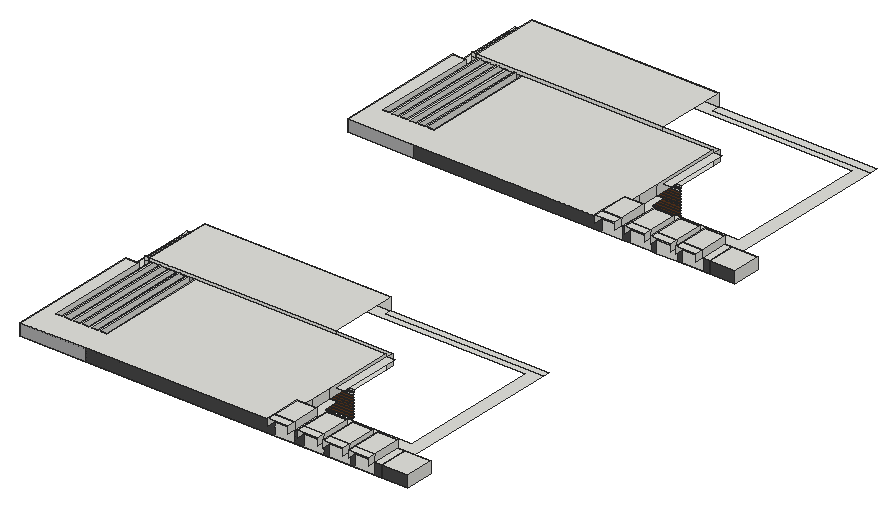
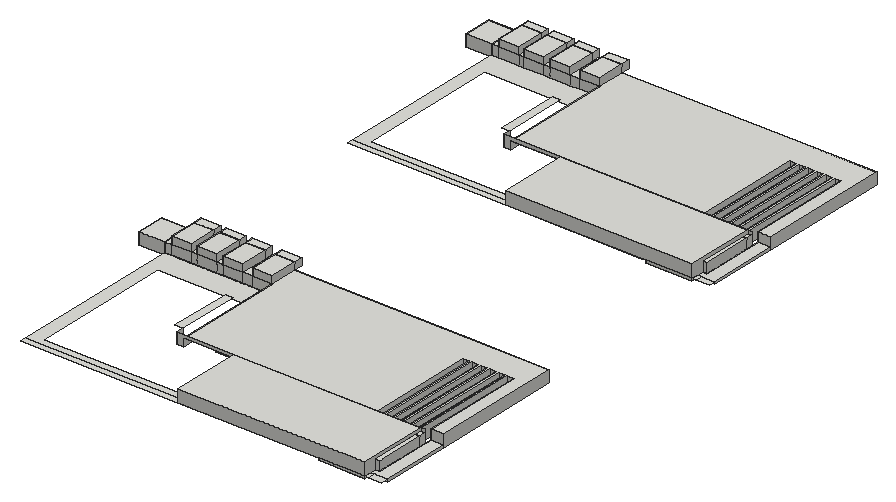
# SketchUp Ruby script. Lengths in inches.
U = 1.inch
M = Sketchup.active_model
def pt(a) = Geom::Point3d.new(a.map { |v| v * U })
def face(e, loops, mat)
  f = e.add_face(loops[0].map { |a| pt(a) })
  loops[1..].each { |l| e.add_face(l.map { |a| pt(a) }).erase! }
  f.material = f.back_material = mat if mat
  f
end
# faces: each face lists its corners as indices into pts; further lists are holes
def faces(e, pts, list, mat = nil) = list.each { |f| face(e, (f[0].is_a?(Array) ? f : [f]).map { |l| l.map { |i| pts[i] } }, mat) }
# xy, xz, yz: faces in a plane at the given z, y or x. An outline is a flat list of corners, or four numbers for a rectangle; further outlines are holes
def ring(l) = l.size == 4 ? [[l[0], l[1]], [l[2], l[1]], [l[2], l[3]], [l[0], l[3]]] : l.each_slice(2).to_a
def flat(e, list, mat, &to3) = list.each { |f| face(e, (f[0].is_a?(Array) ? f : [f]).map { |l| ring(l).map { |u, v| to3.(u, v) } }, mat) }
def xy(e, z, list, mat = nil) = flat(e, list, mat) { |x, y| [x, y, z] }
def xz(e, y, list, mat = nil) = flat(e, list, mat) { |x, z| [x, y, z] }
def yz(e, x, list, mat = nil) = flat(e, list, mat) { |y, z| [x, y, z] }
def lines(e, pts, list) = list.each { |a, b| e.add_line(pt(pts[a]), pt(pts[b])) }
# prism: a flat outline (further loops are holes) pulled along v
def prism(e, loops, v, mat = nil)
  f = face(e, loops, mat); d = Geom::Vector3d.new(v.map { |x| x * U })
  f.pushpull(f.normal.samedirection?(d) ? d.length : -d.length)
end
def box(e, o, s, mat = nil) = prism(e, [[o, [o[0] + s[0], o[1], o[2]], [o[0] + s[0], o[1] + s[1], o[2]], [o[0], o[1] + s[1], o[2]]]], [0, 0, s[2]], mat)
def at(x, y, z, deg = 0) = Geom::Transformation.translation(pt([x, y, z])) * Geom::Transformation.rotation(ORIGIN, Z_AXIS, deg.degrees)
def axes(o, x, y, z) = Geom::Transformation.new([*x, 0, *y, 0, *z, 0, *pt(o).to_a, 1])
def part(name) = M.definitions.add(name)
# library, detail: a bought-in or finely detailed component or shape, given as its bounding box
def library(name, o, s) = part(name).tap { |d| box(d.entities, o, s) }
def detail(e, o, s) = box(e.add_group.entities, o, s)
def put(e, d, t, mat = nil) = e.add_instance(d, t).tap { |i| i.material = mat if mat }
def group(e, t, mat = nil) = e.add_group.tap { |g| g.transformation = t; g.material = mat if mat }.entities
root = M.entities
M.materials.add("[Color M03]1").color = [170, 170, 170]
M.materials.add("[Color M05]").color = [68, 68, 68]
M.materials.add("[Granite Dark Gray]").color = [69, 68, 68]
M.materials.add("[Wood Veneer 01]").color = [96, 56, 29]
c1 = library("A$C06767DEF\#1",[-8.3,1.21,0],[7.09,7.09,5.51])
xy(root,437.47,[[534.24,466.33,620.86,468.64]])
xy(root,437.84,[[533.89,1125.42,620.51,1127.73]])
xy(root,438.5,[[534.24,466.33,620.86,468.64]])
xy(root,438.875,[[533.89,1125.42,620.51,1127.73]])
xy(root,441.53,[[534.24,466.33,620.86,468.64]])
xy(root,441.91,[[533.89,1125.42,620.51,1127.73]])
xy(root,442.5625,[[534.24,466.33,620.86,468.64]])
xy(root,442.9375,[[533.89,1125.42,620.51,1127.73]])
xy(root,445.59,[[534.24,466.33,620.86,468.64]])
xy(root,445.97,[[533.89,1125.42,620.51,1127.73]])
xy(root,446.625,[[534.24,466.33,620.86,468.64]])
xy(root,447,[[533.89,1125.42,620.51,1127.73]])
xy(root,449.66,[[534.24,466.33,620.86,468.64]])
xy(root,450.03,[[533.89,1125.42,620.51,1127.73]])
xy(root,450.6875,[[534.24,466.33,620.86,468.64]])
xy(root,451.0625,[[533.89,1125.42,620.51,1127.73]])
xy(root,453.72,[[534.24,466.33,620.86,468.64]])
xy(root,454.09,[[533.89,1125.42,620.51,1127.73]])
xy(root,454.75,[[534.24,466.33,620.86,468.64]])
xy(root,455.125,[[533.89,1125.42,620.51,1127.73]])
xy(root,457.78,[[534.24,466.33,620.86,468.64]])
xy(root,458.16,[[533.89,1125.42,620.51,1127.73]])
xy(root,458.8125,[[534.24,466.33,620.86,468.64]])
xy(root,459.1875,[[533.89,1125.42,620.51,1127.73]])
xy(root,461.84,[[534.24,466.33,620.86,468.64]])
xy(root,462.22,[[533.89,1125.42,620.51,1127.73]])
xy(root,462.875,[[534.24,466.33,620.86,468.64]])
xy(root,463.25,[[533.89,1125.42,620.51,1127.73]])
xy(root,465.91,[[534.24,466.33,620.86,468.64]])
xy(root,466.28,[[533.89,1125.42,620.51,1127.73]])
xy(root,466.9375,[[534.24,466.33,620.86,468.64]])
xy(root,467.3125,[[533.89,1125.42,620.51,1127.73]])
xy(root,469.97,[[534.24,466.33,620.86,468.64]])
xy(root,470.34,[[533.89,1125.42,620.51,1127.73]])
xy(root,471,[[534.24,466.33,620.86,468.64]])
xy(root,471.375,[[533.89,1125.42,620.51,1127.73]])
xy(root,471.94,[[782.78,322.97,824.53,368.59],[534.24,466.33,609.34,468.64],[228.06,647.98,302.29,659.09]])
xy(root,471.94,[[[200.03,322.97,200.03,647.98,221.15,647.98,221.15,546.92,220.86,546.92,220.86,368.83,230.73,368.83,230.73,556.89,228.06,556.89,228.06,557.39,221.15,557.39,221.15,637.97,228.06,637.97,228.06,647.98,302.29,647.98,302.29,546.92,292.42,546.92,292.42,368.83,302.29,368.83,302.29,340.27,305.19,322.97],[278.11,368.83,287.98,557.39],[263.79,368.83,273.67,557.39],[249.48,368.83,259.36,557.39],[235.17,368.83,245.04,557.39]]],"[Color M03]1")
xy(root,471.94,[[305.19,322.97,302.29,340.27,782.78,340.27,782.78,322.97]],"[Color M05]")
xy(root,474.03,[[609.34,466.33,620.86,468.64]])
xy(root,474.41,[[533.89,1125.42,620.51,1127.73]])
xy(root,475.4375,[[533.89,1125.42,620.51,1127.73]])
xy(root,475.57,[[302.29,340.27,302.29,637.97,308.65,637.97,308.65,534.98,534.24,534.98,534.24,466.33,609.34,466.33,609.34,368.59,782.78,368.59,782.78,340.27],[609.34,368.59,782.78,368.59,782.78,647.98,528.37,647.98,528.37,659.09,308.65,659.09,308.65,637.97,761.66,637.97,761.66,408.96,620.86,408.96,620.86,433.78,609.34,433.78],[200.03,534.98,220.86,534.98,220.86,546.92,221.15,546.92,221.15,637.97,302.29,637.97,302.29,647.98,200.03,647.98],[302.29,637.97,308.65,647.98],[200.03,647.98,221.15,659.09],
  [221.15,647.98,228.06,659.09],[228.06,647.98,302.29,659.09],[302.29,647.98,308.65,659.09],[528.37,647.98,782.78,659.09]])
xy(root,476.38,[[782.4375,982.06,824.1875,1027.68],[533.89,1125.42,609,1127.73],[227.71,1307.07,301.95,1318.18]])
xy(root,476.38,[[[199.6875,982.06,199.6875,1307.07,220.81,1307.07,220.81,1206.01,220.51,1206.01,220.51,1027.92,230.39,1027.92,230.39,1215.98,227.71,1215.98,227.71,1216.48,220.81,1216.48,220.81,1297.06,227.71,1297.06,227.71,1307.07,301.95,1307.07,301.95,1206.01,292.07,1206.01,292.07,1027.92,301.95,1027.92,301.95,999.36,304.85,982.06],[277.76,1027.92,287.64,1216.48],[263.45,1027.92,273.32,1216.48],[249.14,1027.92,259.01,1216.48],[234.82,1027.92,244.7,1216.48]]],"[Color M03]1")
xy(root,476.38,[[304.85,982.06,301.95,999.36,782.4375,999.36,782.4375,982.06]],"[Color M05]")
xy(root,478.09,[[609.34,468.64,620.86,546.92]])
xy(root,478.47,[[609,1125.42,620.51,1127.73]])
xy(root,480,[[301.95,999.36,301.95,1297.06,308.31,1297.06,308.31,1194.07,533.89,1194.07,533.89,1125.42,609,1125.42,609,1027.68,782.4375,1027.68,782.4375,999.36],[609,1027.68,782.4375,1027.68,782.4375,1307.07,528.02,1307.07,528.02,1318.18,308.31,1318.18,308.31,1297.06,761.32,1297.06,761.32,1068.05,620.51,1068.05,620.51,1092.87,609,1092.87],[199.6875,1194.07,220.51,1194.07,220.51,1206.01,220.81,1206.01,220.81,1297.06,301.95,1297.06,301.95,1307.07,199.6875,1307.07],[301.95,1297.06,308.31,1307.07],[199.6875,1307.07,220.81,1318.18],
  [220.81,1307.07,227.71,1318.18],[227.71,1307.07,301.95,1318.18],[301.95,1307.07,308.31,1318.18],[528.02,1307.07,782.4375,1318.18]])
xy(root,482.53,[[609,1127.73,620.51,1206.01]])
xy(root,491.07,[[200.03,322.97,609.34,322.97,609.34,546.92,302.29,546.92,302.29,368.83,292.42,368.83,292.42,546.92,287.98,546.92,287.98,368.83,278.11,368.83,278.11,546.92,273.67,546.92,273.67,368.83,263.79,368.83,263.79,546.92,259.36,546.92,259.36,368.83,249.48,368.83,249.48,546.92,245.04,546.92,245.04,368.83,235.17,368.83,235.17,546.92,230.73,546.92,230.73,368.83,220.86,368.83,220.86,534.98,200.03,534.98],[609.34,322.97,641.55,368.59],[641.55,322.97,657.03,368.59],[657.03,322.97,689.24,368.59],[689.24,322.97,698.65,368.59],
  [698.65,322.97,730.86,368.59],[730.86,322.97,739.28,368.59],[739.28,322.97,771.49,368.59],[771.49,322.97,782.78,368.59],[782.78,322.97,824.53,368.59],
  [221.15,546.92,228.06,557.39],[228.06,546.92,230.73,556.89],[235.17,546.92,245.04,557.39],[249.48,546.92,259.36,557.39],[263.79,546.92,273.67,557.39],
  [278.11,546.92,287.98,557.39],[228.06,556.89,230.73,572.79],[221.15,557.39,228.06,637.97]])
xy(root,495.5,[[199.6875,982.06,609,982.06,609,1206.01,301.95,1206.01,301.95,1027.92,292.07,1027.92,292.07,1206.01,287.64,1206.01,287.64,1027.92,277.76,1027.92,277.76,1206.01,273.32,1206.01,273.32,1027.92,263.45,1027.92,263.45,1206.01,259.01,1206.01,259.01,1027.92,249.14,1027.92,249.14,1206.01,244.7,1206.01,244.7,1027.92,234.82,1027.92,234.82,1206.01,230.39,1206.01,230.39,1027.92,220.51,1027.92,220.51,1194.07,199.6875,1194.07],[609,982.06,641.2,1027.68],[641.2,982.06,656.68,1027.68],[656.68,982.06,688.89,1027.68],[688.89,982.06,698.31,1027.68],
  [698.31,982.06,730.52,1027.68],[730.52,982.06,738.93,1027.68],[738.93,982.06,771.14,1027.68],[771.14,982.06,782.4375,1027.68],[782.4375,982.06,824.1875,1027.68],
  [220.81,1206.01,227.71,1216.48],[227.71,1206.01,230.39,1215.98],[234.82,1206.01,244.7,1216.48],[249.14,1206.01,259.01,1216.48],[263.45,1206.01,273.32,1216.48],
  [277.76,1206.01,287.64,1216.48],[227.71,1215.98,230.39,1231.88],[220.81,1216.48,227.71,1297.06]])
xy(root,496.07,[[620.86,433.78,632.79,534.98],[228.06,546.92,528.37,659.09]])
xy(root,500.5,[[620.51,1092.87,632.45,1194.07],[227.71,1206.01,528.02,1318.18]])
xy(root,502.82,[[609.34,309.65,641.55,322.97],[657.03,309.65,689.24,322.97],[698.65,309.65,730.86,322.97],[739.28,309.65,771.49,322.97],[609.34,322.97,641.55,368.59],
  [657.03,322.97,689.24,368.59],[698.65,322.97,730.86,368.59],[739.28,322.97,771.49,368.59]])
xy(root,507.25,[[609,968.74,641.2,982.06],[656.68,968.74,688.89,982.06],[698.31,968.74,730.52,982.06],[738.93,968.74,771.14,982.06],[609,982.06,641.2,1027.68],
  [656.68,982.06,688.89,1027.68],[698.31,982.06,730.52,1027.68],[738.93,982.06,771.14,1027.68]])
xz(root,322.97,[[609.34,471.94,641.55,491.07],[657.03,471.94,689.24,491.07],[698.65,471.94,730.86,491.07],[739.28,471.94,771.49,491.07],[609.34,491.07,641.55,502.82],
  [657.03,491.07,689.24,502.82],[698.65,491.07,730.86,502.82],[739.28,491.07,771.49,502.82]])
xz(root,322.97,[[200.03,471.94,305.19,491.07]],"[Color M03]1")
xz(root,322.97,[[305.19,471.94,609.34,491.07],[641.55,471.94,657.03,491.07],[689.24,471.94,698.65,491.07],[730.86,471.94,739.28,491.07],[771.49,471.94,782.78,491.07],
  [782.78,471.94,824.53,491.07]],"[Granite Dark Gray]")
xz(root,340.27,[[302.29,471.94,782.78,475.57]])
xz(root,368.59,[[782.78,471.94,824.53,491.07],[609.34,475.57,641.55,491.07],[641.55,475.57,657.03,491.07],[657.03,475.57,689.24,491.07],[689.24,475.57,698.65,491.07],
  [698.65,475.57,730.86,491.07],[730.86,475.57,739.28,491.07],[739.28,475.57,771.49,491.07],[771.49,475.57,782.78,491.07],[609.34,491.07,641.55,502.82],
  [657.03,491.07,689.24,502.82],[698.65,491.07,730.86,502.82],[739.28,491.07,771.49,502.82]])
xz(root,368.83,[[220.86,471.94,230.73,491.07],[235.17,471.94,245.04,491.07],[249.48,471.94,259.36,491.07],[263.79,471.94,273.67,491.07],[278.11,471.94,287.98,491.07],
  [292.42,471.94,302.29,491.07]])
xz(root,466.33,[[534.24,471,620.86,471,620.86,474.03,609.34,474.03,609.34,471.94,534.24,471.94]])
xz(root,466.33,[[534.24,438.5,620.86,441.53],[534.24,442.5625,620.86,445.59],[534.24,446.625,620.86,449.66],[534.24,450.6875,620.86,453.72],[534.24,454.75,620.86,457.78],
  [534.24,458.8125,620.86,461.84],[534.24,462.875,620.86,465.91],[534.24,466.9375,620.86,469.97],[534.24,471.94,609.34,475.57]],"[Wood Veneer 01]")
xz(root,468.64,[[534.24,437.47,620.86,438.5],[534.24,441.53,620.86,442.5625],[534.24,445.59,620.86,446.625],[534.24,449.66,620.86,450.6875],[534.24,453.72,620.86,454.75],
  [534.24,457.78,620.86,458.8125],[534.24,461.84,620.86,462.875],[534.24,465.91,620.86,466.9375],[534.24,469.97,620.86,471],[534.24,471.94,609.34,474.03],
  [609.34,474.03,620.86,475.0625],[534.24,475.0625,609.34,478.09],[609.34,475.0625,620.86,478.09]])
xz(root,534.98,[[200.03,475.57,220.86,491.07]])
xz(root,546.92,[[220.86,471.94,221.15,475.57],[609.34,478.09,609.34,491.07,528.37,491.07,528.37,496.07,620.86,496.07,620.86,478.09],[221.15,491.07,228.06,496.07],[228.06,491.07,528.37,496.07]])
xz(root,546.92,[[292.42,471.94,302.29,491.07]],"[Color M03]1")
xz(root,556.89,[[228.06,471.94,230.73,491.07]])
xz(root,557.39,[[221.15,471.82,228.06,471.94]])
xz(root,557.39,[[221.15,471.94,228.06,491.07],[235.17,471.94,245.04,491.07],[249.48,471.94,259.36,491.07],[263.79,471.94,273.67,491.07],[278.11,471.94,287.98,491.07]],"[Color M03]1")
xz(root,637.97,[[221.15,471.82,228.06,471.94],[221.15,471.94,228.06,475.57],[221.15,475.57,228.06,491.07]])
xz(root,647.98,[[228.06,471.94,302.29,475.57]])
xz(root,659.09,[[228.06,471.94,302.29,475.57],[228.06,475.57,528.37,496.07]])
xz(root,982.06,[[609,476.38,641.2,495.5],[656.68,476.38,688.89,495.5],[698.31,476.38,730.52,495.5],[738.93,476.38,771.14,495.5],[609,495.5,641.2,507.25],
  [656.68,495.5,688.89,507.25],[698.31,495.5,730.52,507.25],[738.93,495.5,771.14,507.25]])
xz(root,982.06,[[199.6875,476.38,304.85,495.5]],"[Color M03]1")
xz(root,982.06,[[304.85,476.38,609,495.5],[641.2,476.38,656.68,495.5],[688.89,476.38,698.31,495.5],[730.52,476.38,738.93,495.5],[771.14,476.38,782.4375,495.5],
  [782.4375,476.38,824.1875,495.5]],"[Granite Dark Gray]")
xz(root,999.36,[[301.95,476.38,782.4375,480]])
xz(root,1027.68,[[782.4375,476.38,824.1875,495.5],[609,480,641.2,495.5],[641.2,480,656.68,495.5],[656.68,480,688.89,495.5],[688.89,480,698.31,495.5],
  [698.31,480,730.52,495.5],[730.52,480,738.93,495.5],[738.93,480,771.14,495.5],[771.14,480,782.4375,495.5],[609,495.5,641.2,507.25],
  [656.68,495.5,688.89,507.25],[698.31,495.5,730.52,507.25],[738.93,495.5,771.14,507.25]])
xz(root,1027.92,[[220.51,476.38,230.39,495.5],[234.82,476.38,244.7,495.5],[249.14,476.38,259.01,495.5],[263.45,476.38,273.32,495.5],[277.76,476.38,287.64,495.5],
  [292.07,476.38,301.95,495.5]])
xz(root,1125.42,[[533.89,475.4375,620.51,475.4375,620.51,478.47,609,478.47,609,476.38,533.89,476.38]])
xz(root,1125.42,[[533.89,438.875,620.51,441.91],[533.89,442.9375,620.51,445.97],[533.89,447,620.51,450.03],[533.89,451.0625,620.51,454.09],[533.89,455.125,620.51,458.16],
  [533.89,459.1875,620.51,462.22],[533.89,463.25,620.51,466.28],[533.89,467.3125,620.51,470.34],[533.89,471.375,620.51,474.41],[533.89,476.38,609,480]],"[Wood Veneer 01]")
xz(root,1127.73,[[533.89,437.84,620.51,438.875],[533.89,441.91,620.51,442.9375],[533.89,445.97,620.51,447],[533.89,450.03,620.51,451.0625],[533.89,454.09,620.51,455.125],
  [533.89,458.16,620.51,459.1875],[533.89,462.22,620.51,463.25],[533.89,466.28,620.51,467.3125],[533.89,470.34,620.51,471.375],[533.89,474.41,620.51,475.4375],
  [533.89,476.38,609,478.47],[609,478.47,620.51,479.5],[533.89,479.5,609,482.53],[609,479.5,620.51,482.53]])
xz(root,1194.07,[[199.6875,480,220.51,495.5]])
xz(root,1206.01,[[220.51,476.38,220.81,480],[609,482.53,609,495.5,528.02,495.5,528.02,500.5,620.51,500.5,620.51,482.53],[220.81,495.5,227.71,500.5],[227.71,495.5,528.02,500.5]])
xz(root,1206.01,[[292.07,476.38,301.95,495.5]],"[Color M03]1")
xz(root,1215.98,[[227.71,476.38,230.39,495.5]])
xz(root,1216.48,[[220.81,476.25,227.71,476.38]])
xz(root,1216.48,[[220.81,476.38,227.71,495.5],[234.82,476.38,244.7,495.5],[249.14,476.38,259.01,495.5],[263.45,476.38,273.32,495.5],[277.76,476.38,287.64,495.5]],"[Color M03]1")
xz(root,1297.06,[[220.81,476.25,227.71,476.38],[220.81,476.38,227.71,480],[220.81,480,227.71,495.5]])
xz(root,1307.07,[[227.71,476.38,301.95,480]])
xz(root,1318.18,[[227.71,476.38,301.95,480],[227.71,480,528.02,500.5]])
yz(root,199.6875,[[982.06,476.38,1194.07,495.5],[1194.07,476.38,1307.07,480]])
yz(root,200.03,[[322.97,471.94,534.98,491.07],[534.98,471.94,647.98,475.57]])
yz(root,220.51,[[1027.92,476.38,1206.01,476.38,1206.01,480,1194.07,480,1194.07,495.5,1027.92,495.5]])
yz(root,220.81,[[1216.48,476.25,1297.06,476.38],[1206.01,476.38,1216.48,480],[1216.48,476.38,1297.06,480],[1206.01,480,1216.48,495.5],[1216.48,480,1297.06,495.5]])
yz(root,220.86,[[368.83,471.94,546.92,471.94,546.92,475.57,534.98,475.57,534.98,491.07,368.83,491.07]])
yz(root,221.15,[[557.39,471.82,637.97,471.94],[546.92,471.94,557.39,475.57],[557.39,471.94,637.97,475.57],[546.92,475.57,557.39,491.07],[557.39,475.57,637.97,491.07]])
yz(root,227.71,[[1297.06,476.38,1297.06,495.5,1206.01,495.5,1206.01,500.5,1318.18,500.5,1318.18,480,1307.07,480,1307.07,476.38],[1215.98,476.38,1216.48,495.5],[1307.07,476.38,1318.18,480]])
yz(root,228.06,[[637.97,471.94,637.97,491.07,546.92,491.07,546.92,496.07,659.09,496.07,659.09,475.57,647.98,475.57,647.98,471.94],[556.89,471.94,557.39,491.07],[647.98,471.94,659.09,475.57]])
yz(root,230.39,[[1027.92,476.38,1215.98,495.5]])
yz(root,230.73,[[368.83,471.94,556.89,491.07]])
yz(root,234.82,[[1027.92,476.38,1216.48,495.5]])
yz(root,235.17,[[368.83,471.94,557.39,491.07]])
yz(root,244.7,[[1027.92,476.38,1216.48,495.5]])
yz(root,245.04,[[368.83,471.94,557.39,491.07]])
yz(root,249.14,[[1027.92,476.38,1216.48,495.5]])
yz(root,249.48,[[368.83,471.94,557.39,491.07]])
yz(root,259.01,[[1027.92,476.38,1216.48,495.5]])
yz(root,259.36,[[368.83,471.94,557.39,491.07]])
yz(root,263.45,[[1027.92,476.38,1216.48,495.5]])
yz(root,263.79,[[368.83,471.94,557.39,491.07]])
yz(root,273.32,[[1027.92,476.38,1216.48,495.5]])
yz(root,273.67,[[368.83,471.94,557.39,491.07]])
yz(root,277.76,[[1027.92,476.38,1216.48,495.5]])
yz(root,278.11,[[368.83,471.94,557.39,491.07]])
yz(root,287.64,[[1027.92,476.38,1216.48,495.5]])
yz(root,287.98,[[368.83,471.94,557.39,491.07]])
yz(root,292.07,[[1027.92,476.38,1206.01,495.5]])
yz(root,292.42,[[368.83,471.94,546.92,491.07]])
yz(root,301.95,[[999.36,476.38,1027.92,480],[1206.01,476.38,1307.07,480],[1307.07,476.38,1318.18,480],[1027.92,480,1206.01,495.5]])
yz(root,302.29,[[340.27,471.94,368.83,475.57],[546.92,471.94,647.98,475.57],[647.98,471.94,659.09,475.57],[368.83,475.57,546.92,491.07]])
yz(root,533.89,[[1125.42,476.38,1127.73,480]])
yz(root,534.24,[[466.33,471.94,468.64,475.57]])
yz(root,609,[[1125.42,476.38,1127.73,478.47],[1125.42,478.47,1127.73,478.47,1127.73,482.53,1206.01,482.53,1206.01,495.5,1092.87,495.5,1092.87,480,1125.42,480],[1027.68,480,1056.54,495.5],[1056.54,480,1092.87,495.5],[968.74,495.5,982.06,507.25],
  [982.06,495.5,1027.68,507.25]])
yz(root,609.34,[[466.33,471.94,468.64,474.03],[466.33,474.03,468.64,474.03,468.64,478.09,546.92,478.09,546.92,491.07,433.78,491.07,433.78,475.57,466.33,475.57],[368.59,475.57,397.45,491.07],[397.45,475.57,433.78,491.07],[309.65,491.07,322.97,502.82],
  [322.97,491.07,368.59,502.82]])
yz(root,620.51,[[1194.07,482.53,1206.01,500.5]])
yz(root,620.86,[[534.98,478.09,546.92,496.07]])
yz(root,641.2,[[968.74,495.5,982.06,507.25],[982.06,495.5,1027.68,507.25]])
yz(root,641.55,[[309.65,491.07,322.97,502.82],[322.97,491.07,368.59,502.82]])
yz(root,656.68,[[968.74,495.5,982.06,507.25],[982.06,495.5,1027.68,507.25]])
yz(root,657.03,[[309.65,491.07,322.97,502.82],[322.97,491.07,368.59,502.82]])
yz(root,688.89,[[968.74,495.5,982.06,507.25],[982.06,495.5,1027.68,507.25]])
yz(root,689.24,[[309.65,491.07,322.97,502.82],[322.97,491.07,368.59,502.82]])
yz(root,698.31,[[968.74,495.5,982.06,507.25],[982.06,495.5,1027.68,507.25]])
yz(root,698.65,[[309.65,491.07,322.97,502.82],[322.97,491.07,368.59,502.82]])
yz(root,730.52,[[968.74,495.5,982.06,507.25],[982.06,495.5,1027.68,507.25]])
yz(root,730.86,[[309.65,491.07,322.97,502.82],[322.97,491.07,368.59,502.82]])
yz(root,738.93,[[968.74,495.5,982.06,507.25],[982.06,495.5,1027.68,507.25]])
yz(root,739.28,[[309.65,491.07,322.97,502.82],[322.97,491.07,368.59,502.82]])
yz(root,771.14,[[968.74,495.5,982.06,507.25],[982.06,495.5,1027.68,507.25]])
yz(root,771.49,[[309.65,491.07,322.97,502.82],[322.97,491.07,368.59,502.82]])
yz(root,782.4375,[[982.06,476.38,999.36,476.38,999.36,480,1027.68,480,1027.68,495.5,982.06,495.5],[999.36,476.38,1027.68,480]])
yz(root,782.78,[[322.97,471.94,340.27,471.94,340.27,475.57,368.59,475.57,368.59,491.07,322.97,491.07],[340.27,471.94,368.59,475.57]])
yz(root,824.1875,[[982.06,476.38,1027.68,495.5]])
yz(root,824.53,[[322.97,471.94,368.59,491.07]])
put(root,c1,at(340.86,1092.87,474.49))
put(root,c1,at(341.21,433.78,470.05))
put(root,c1,at(415.49,1092.87,474.49))
put(root,c1,at(415.83,433.78,470.05))
put(root,c1,at(493.68,1092.87,474.49))
put(root,c1,at(494.02,433.78,470.05))
